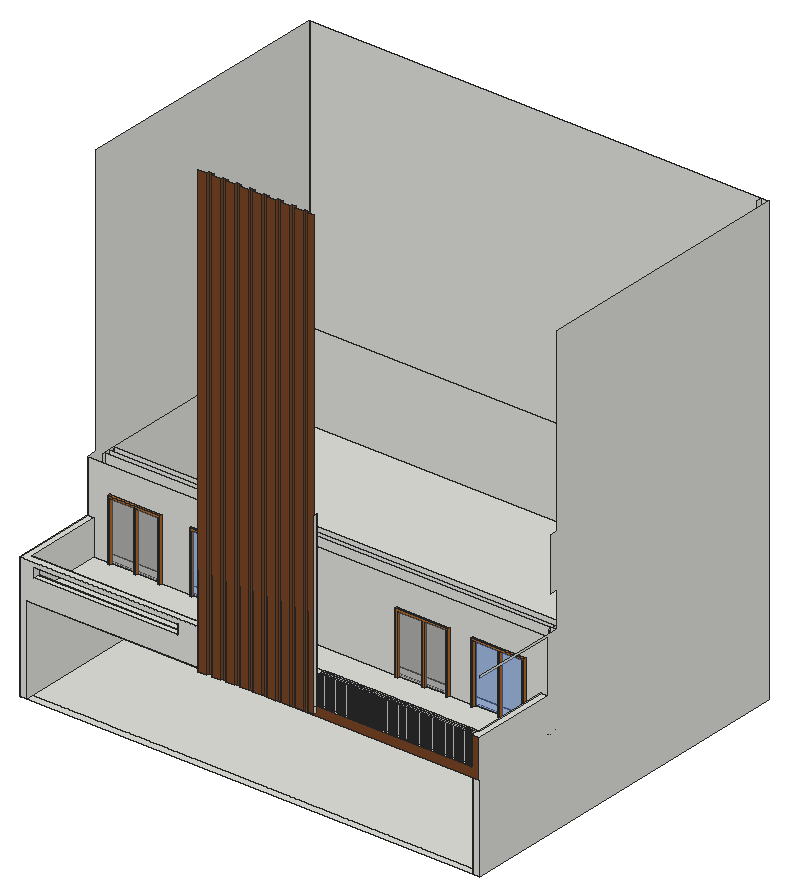
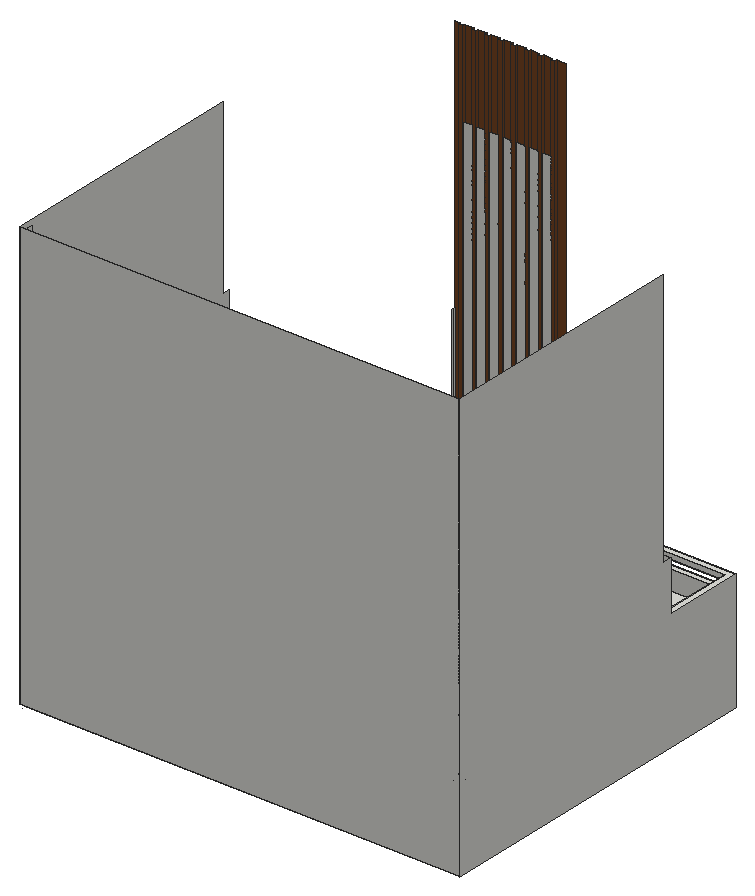
# SketchUp Ruby script. Lengths in inches.
U = 1.inch
M = Sketchup.active_model
def pt(a) = Geom::Point3d.new(a.map { |v| v * U })
def face(e, loops, mat)
  f = e.add_face(loops[0].map { |a| pt(a) })
  loops[1..].each { |l| e.add_face(l.map { |a| pt(a) }).erase! }
  f.material = f.back_material = mat if mat
  f
end
# faces: each face lists its corners as indices into pts; further lists are holes
def faces(e, pts, list, mat = nil) = list.each { |f| face(e, (f[0].is_a?(Array) ? f : [f]).map { |l| l.map { |i| pts[i] } }, mat) }
# xy, xz, yz: faces in a plane at the given z, y or x. An outline is a flat list of corners, or four numbers for a rectangle; further outlines are holes
def ring(l) = l.size == 4 ? [[l[0], l[1]], [l[2], l[1]], [l[2], l[3]], [l[0], l[3]]] : l.each_slice(2).to_a
def flat(e, list, mat, &to3) = list.each { |f| face(e, (f[0].is_a?(Array) ? f : [f]).map { |l| ring(l).map { |u, v| to3.(u, v) } }, mat) }
def xy(e, z, list, mat = nil) = flat(e, list, mat) { |x, y| [x, y, z] }
def xz(e, y, list, mat = nil) = flat(e, list, mat) { |x, z| [x, y, z] }
def yz(e, x, list, mat = nil) = flat(e, list, mat) { |y, z| [x, y, z] }
def lines(e, pts, list) = list.each { |a, b| e.add_line(pt(pts[a]), pt(pts[b])) }
# prism: a flat outline (further loops are holes) pulled along v
def prism(e, loops, v, mat = nil)
  f = face(e, loops, mat); d = Geom::Vector3d.new(v.map { |x| x * U })
  f.pushpull(f.normal.samedirection?(d) ? d.length : -d.length)
end
def box(e, o, s, mat = nil) = prism(e, [[o, [o[0] + s[0], o[1], o[2]], [o[0] + s[0], o[1] + s[1], o[2]], [o[0], o[1] + s[1], o[2]]]], [0, 0, s[2]], mat)
def at(x, y, z, deg = 0) = Geom::Transformation.translation(pt([x, y, z])) * Geom::Transformation.rotation(ORIGIN, Z_AXIS, deg.degrees)
def axes(o, x, y, z) = Geom::Transformation.new([*x, 0, *y, 0, *z, 0, *pt(o).to_a, 1])
def part(name) = M.definitions.add(name)
# library, detail: a bought-in or finely detailed component or shape, given as its bounding box
def library(name, o, s) = part(name).tap { |d| box(d.entities, o, s) }
def detail(e, o, s) = box(e.add_group.entities, o, s)
def put(e, d, t, mat = nil) = e.add_instance(d, t).tap { |i| i.material = mat if mat }
def group(e, t, mat = nil) = e.add_group.tap { |g| g.transformation = t; g.material = mat if mat }.entities
root = M.entities
M.materials.add("[Translucent Glass Blue]").color = [100, 149, 237]
M.materials["[Translucent Glass Blue]"].alpha = 0.5
M.materials.add("[Translucent Glass Gray]").color = [128, 128, 128]
M.materials["[Translucent Glass Gray]"].alpha = 0.5
M.materials.add("[Wood Bamboo]").color = [177, 105, 43]
M.materials.add("[Wood Veneer 01]").color = [120, 70, 37]
xy(root,0,[[0,6,1.4375,499.375],[1.4375,6,2.375,499.375],[2.375,6,2.375,499.375,620.5,499.375,620.5,490.375,9,490.375,9,6],[9,6,620.5,15],[620.5,6,620.75,497.0625],
  [620.75,6,628.8125,490.375],[628.8125,6,629.5625,499.375],[629.5625,6,630,499.375],[9,15,620.5,490.375],[620.75,490.375,628.8125,499.375],
  [620.5,497.0625,620.75,499.3125],[620.5,499.3125,620.75,499.375]])
xy(root,120,[[248.625,0,248.625,6,406.875,6,406.875,3,261.1,3,261.1,0],[406.875,3,406.875,6,9,6,9,490.375,620.5,490.375,620.5,3],[620.5,3,630,6]])
xy(root,120.375,[[267.4375,0,279.91,3]])
xy(root,120.75,[[286.25,0,298.72,3]])
xy(root,121.125,[[305.06,0,317.53,3]])
xy(root,121.5,[[323.87,0,336.34,3]])
xy(root,121.875,[[342.68,0,355.16,3]])
xy(root,122.0625,[[621,125.83,628.8125,136.3125]])
xy(root,122.25,[[361.49,0,373.97,3]])
xy(root,122.625,[[380.31,0,392.78,3]])
xy(root,123,[[399.12,0,406.875,3],[9,15,621,15,621,121.57,599.4,121.57,599.4,118.57,596.4,118.57,596.4,121.57,567.09,121.57,567.09,118.57,563.4,118.57,563.4,123.19,530.4,123.19,530.4,118.57,527.4,118.57,527.4,121.57,495.49,121.57,495.49,118.57,492.49,118.57,492.49,121.57,463.62,121.57,463.62,118.57,459.49,118.57,459.49,121.57,426.49,121.57,426.49,118.57,423.49,118.57,423.49,121.57,213.64,121.57,213.64,118.57,210.64,118.57,210.64,121.57,180.6,121.57,180.6,118.57,177.64,118.57,177.64,121.57,144.64,121.57,144.64,118.57,141.64,118.57,141.64,121.57,101.8,121.57,101.8,118.57,98.8,118.57,98.8,121.57,68.43,121.57,68.43,118.57,65.8,118.57,65.8,121.57,32.8,121.57,32.8,118.57,29.8,118.57,29.8,121.57,9,121.57],[423.49,118.57,426.49,121.57],[459.49,118.57,463.62,121.57],[492.49,118.57,495.49,121.57],
  [527.4,118.57,530.4,121.57],[563.4,118.57,567.09,121.57],[596.4,118.57,599.4,121.57],[620.5,121.57,621,125.58],[0,125.58,619.6875,125.83],
  [619.6875,125.58,620.5,125.83],[620.5,125.58,621,125.83],[621,125.58,628.8125,125.83],[620.5,125.83,621,135.01],[621,125.83,628.8125,135.01],
  [620.5,135.01,621,136.3125],[621,135.01,628.8125,136.3125],[620.5,136.3125,621,139.19],[9,139.19,620.5,146.07],[620.5,139.19,621,146.07],
  [9,146.07,620.5,155.08],[620.5,146.07,621,155.08],[9,155.08,621,490.375]])
xy(root,123.125,[[621,125.83,628.8125,135.01],[621,135.01,628.8125,136.3125]])
xy(root,132.4,[[406.875,3,620.5,3,620.5,6,618.8,6,618.8,15,617.26,15,617.26,6,615.74,6,615.74,15,614.19,15,614.19,6,612.68,6,612.68,15,611.13,15,611.13,6,609.62,6,609.62,15,608.07,15,608.07,6,606.55,6,606.55,15,605.01,15,605.01,6,603.49,6,603.49,15,601.94,15,601.94,6,600.43,6,600.43,15,598.88,15,598.88,6,597.37,6,597.37,15,595.82,15,595.82,6.5,594.3,6.5,594.3,15,592.76,15,592.76,6,590.74,6,590.74,15,589.19,15,589.19,6,587.18,6,587.18,15,585.63,15,585.63,6,583.62,6,583.62,15,582.07,15,582.07,6,580.05,6,580.05,15,578.51,15,578.51,6,576.49,6,576.49,15,574.94,15,574.94,6,572.93,6,572.93,15,571.38,15,571.38,6,569.37,6,569.37,15,567.82,15,567.82,6,565.8,6,565.8,15,564.26,15,564.26,6,562.24,6,562.24,15,560.69,15,560.69,6,558.68,6,558.68,15,557.13,15,557.13,6,555.12,6,555.12,15,553.57,15,553.57,6,551.55,6,551.55,15,550.01,15,550.01,6,547.99,6,547.99,15,546.44,15,546.44,6,544.43,6,544.43,15,542.88,15,542.88,6,540.87,6,540.87,15,539.32,15,539.32,6,537.3,6,537.3,15,535.76,15,535.76,6,533.74,6,533.74,15,532.19,15,532.19,6,530.18,6,530.18,15,528.63,15,528.63,6,526.62,6,526.62,15,525.07,15,525.07,6,523.05,6,523.05,15,521.51,15,521.51,6,519.3,6,519.3,15,517.76,15,517.76,6,515.55,6,515.55,15,514.01,15,514.01,6,511.8,6,511.8,15,510.26,15,510.26,6,508.05,6,508.05,15,506.51,15,506.51,6,504.3,6,504.3,15,502.76,15,502.76,6,500.55,6,500.55,15,499.01,15,499.01,6,496.8,6,496.8,15,495.26,15,495.26,6,493.05,6,493.05,15,491.51,15,491.51,6,489.3,6,489.3,15,487.76,15,487.76,6,485.55,6,485.55,15,484.01,15,484.01,6,481.8,6,481.8,15,480.26,15,480.26,6,478.05,6,478.05,15,476.51,15,476.51,6,474.3,6,474.3,15,472.76,15,472.76,6,470.55,6,470.55,15,469.01,15,469.01,6,466.8,6,466.8,15,465.26,15,465.26,6,463.05,6,463.05,15,461.51,15,461.51,6,459.3,6,459.3,15,457.76,15,457.76,6,455.55,6,455.55,15,454.01,15,454.01,6,451.8,6,451.8,15,450.26,15,450.26,6,448.05,6,448.05,15,446.51,15,446.51,6,444.3,6,444.3,15,442.76,15,442.76,6,440.55,6,440.55,15,439.01,15,439.01,6,436.8,6,436.8,15,435.26,15,435.26,6,433.05,6,433.05,15,431.51,15,431.51,6,429.3,6,429.3,15,427.76,15,427.76,6,425.55,6,425.55,15,424.01,15,424.01,6,421.8,6,421.8,15,420.26,15,420.26,6,418.05,6,418.05,15,416.51,15,416.51,6,414.3,6,414.3,15,412.76,15,412.76,6,410.55,6,410.55,15,409.01,15,409.01,6,406.875,6]])
xy(root,150.64,[[18.24,6,215.68,15]])
xy(root,164.2,[[18.24,6,215.68,15]])
xy(root,171,[[620.5,3,630,3,630,121.92,621,121.57,621,15,618.8,15,618.8,6,620.5,6],[0,6,409.01,6,409.01,15,9,15,9,121.57,0,121.57],[410.55,6,412.76,15],[414.3,6,416.51,15],[418.05,6,420.26,15],
  [421.8,6,424.01,15],[425.55,6,427.76,15],[429.3,6,431.51,15],[433.05,6,435.26,15],[436.8,6,439.01,15],
  [440.55,6,442.76,15],[444.3,6,446.51,15],[448.05,6,450.26,15],[451.8,6,454.01,15],[455.55,6,457.76,15],
  [459.3,6,461.51,15],[463.05,6,465.26,15],[466.8,6,469.01,15],[470.55,6,472.76,15],[474.3,6,476.51,15],
  [478.05,6,480.26,15],[481.8,6,484.01,15],[485.55,6,487.76,15],[489.3,6,491.51,15],[493.05,6,495.26,15],
  [496.8,6,499.01,15],[500.55,6,502.76,15],[504.3,6,506.51,15],[508.05,6,510.26,15],[511.8,6,514.01,15],
  [515.55,6,517.76,15],[519.3,6,521.51,15],[523.05,6,525.07,15],[526.62,6,528.63,15],[530.18,6,532.19,15],
  [533.74,6,535.76,15],[537.3,6,539.32,15],[540.87,6,542.88,15],[544.43,6,546.44,15],[547.99,6,550.01,15],
  [551.55,6,553.57,15],[555.12,6,557.13,15],[558.68,6,560.69,15],[562.24,6,564.26,15],[565.8,6,567.82,15],
  [569.37,6,571.38,15],[572.93,6,574.94,15],[576.49,6,578.51,15],[580.05,6,582.07,15],[583.62,6,585.63,15],
  [587.18,6,589.19,15],[590.74,6,592.76,15],[597.37,6,598.88,15],[600.43,6,601.94,15],[603.49,6,605.01,15],
  [606.55,6,608.07,15],[609.62,6,611.13,15],[612.68,6,614.19,15],[615.74,6,617.26,15],[594.3,6.5,595.82,15]])
xy(root,204,[[32.8,118.57,65.8,121.57],[68.43,118.57,98.8,121.57],[144.64,118.57,177.64,121.57],[180.6,118.57,210.64,121.57],[426.49,118.57,459.49,121.57],
  [463.62,118.57,492.49,121.57],[530.4,118.57,563.4,121.57],[567.09,118.57,596.4,121.57],[530.4,121.57,563.4,123.19]],"[Wood Bamboo]")
xy(root,207,[[29.8,118.57,101.8,121.57],[141.64,118.57,213.64,121.57],[423.49,118.57,495.49,121.57],[527.4,118.57,599.4,121.57]],"[Wood Bamboo]")
xz(root,0,[[248.625,120,261.1,735.4375],[267.4375,120.375,279.91,735.4375],[286.25,120.75,298.72,735.4375],[305.06,121.125,317.53,735.4375],[323.87,121.5,336.34,735.4375],
  [342.68,121.875,355.16,735.4375],[361.49,122.25,373.97,735.4375],[380.31,122.625,392.78,735.21],[399.12,123,406.875,735.4375]],"[Wood Veneer 01]")
xz(root,3,[[267.4375,120.375,279.91,612],[286.25,120.75,298.72,612],[305.06,121.125,317.53,612],[323.87,121.5,336.34,612],[342.68,121.875,355.16,612],
  [361.49,122.25,373.97,612],[380.31,122.625,392.78,612]])
xz(root,3,[[261.1,120,630,120,630,171,620.5,171,620.5,132.4,406.875,132.4,406.875,123,399.12,123,399.12,735.4375,392.78,735.4375,392.78,122.625,380.31,122.625,380.31,735.4375,373.97,735.4375,373.97,122.25,361.49,122.25,361.49,735.4375,355.16,735.4375,355.16,121.875,342.68,121.875,342.68,735.4375,336.34,735.4375,336.34,121.5,323.87,121.5,323.87,735.4375,317.53,735.4375,317.53,121.125,305.06,121.125,305.06,735.4375,298.72,735.4375,298.72,120.75,286.25,120.75,286.25,735.4375,279.91,735.4375,279.91,120.375,267.4375,120.375,267.4375,735.4375,261.1,735.4375]],"[Wood Veneer 01]")
xz(root,6,[[[0,0,9,0,9,120,248.625,120,248.625,171,0,171],[18.24,150.64,215.68,164.2]],[620.5,0,630,120],[248.625,120,406.875,123],[248.625,123,406.875,171],[406.875,132.4,409.01,171],
  [410.55,132.4,412.76,171],[414.3,132.4,416.51,171],[418.05,132.4,420.26,171],[421.8,132.4,424.01,171],[425.55,132.4,427.76,171],
  [429.3,132.4,431.51,171],[433.05,132.4,435.26,171],[436.8,132.4,439.01,171],[440.55,132.4,442.76,171],[444.3,132.4,446.51,171],
  [448.05,132.4,450.26,171],[451.8,132.4,454.01,171],[455.55,132.4,457.76,171],[459.3,132.4,461.51,171],[463.05,132.4,465.26,171],
  [466.8,132.4,469.01,171],[470.55,132.4,472.76,171],[474.3,132.4,476.51,171],[478.05,132.4,480.26,171],[481.8,132.4,484.01,171],
  [485.55,132.4,487.76,171],[489.3,132.4,491.51,171],[493.05,132.4,495.26,171],[496.8,132.4,499.01,171],[500.55,132.4,502.76,171],
  [504.3,132.4,506.51,171],[508.05,132.4,510.26,171],[511.8,132.4,514.01,171],[515.55,132.4,517.76,171],[519.3,132.4,521.51,171],
  [523.05,132.4,525.07,171],[526.62,132.4,528.63,171],[530.18,132.4,532.19,171],[533.74,132.4,535.76,171],[537.3,132.4,539.32,171],
  [540.87,132.4,542.88,171],[544.43,132.4,546.44,171],[547.99,132.4,550.01,171],[551.55,132.4,553.57,171],[555.12,132.4,557.13,171],
  [558.68,132.4,560.69,171],[562.24,132.4,564.26,171],[565.8,132.4,567.82,171],[569.37,132.4,571.38,171],[572.93,132.4,574.94,171],
  [576.49,132.4,578.51,171],[580.05,132.4,582.07,171],[583.62,132.4,585.63,171],[587.18,132.4,589.19,171],[590.74,132.4,592.76,171],
  [597.37,132.4,598.88,171],[600.43,132.4,601.94,171],[603.49,132.4,605.01,171],[606.55,132.4,608.07,171],[609.62,132.4,611.13,171],
  [612.68,132.4,614.19,171],[615.74,132.4,617.26,171],[618.8,132.4,620.32,171],[620.32,132.4,620.5,171],[248.625,171,406.875,243]])
xz(root,6.5,[[594.3,132.4,595.82,171]])
xz(root,15,[[620.5,122.75,621,122.9375],[620.5,122.9375,621,123],[[9,123,9,171,409.01,171,409.01,132.4,410.55,132.4,410.55,171,412.76,171,412.76,132.4,414.3,132.4,414.3,171,416.51,171,416.51,132.4,418.05,132.4,418.05,171,420.26,171,420.26,132.4,421.8,132.4,421.8,171,424.01,171,424.01,132.4,425.55,132.4,425.55,171,427.76,171,427.76,132.4,429.3,132.4,429.3,171,431.51,171,431.51,132.4,433.05,132.4,433.05,171,435.26,171,435.26,132.4,436.8,132.4,436.8,171,439.01,171,439.01,132.4,440.55,132.4,440.55,171,442.76,171,442.76,132.4,444.3,132.4,444.3,171,446.51,171,446.51,132.4,448.05,132.4,448.05,171,450.26,171,450.26,132.4,451.8,132.4,451.8,171,454.01,171,454.01,132.4,455.55,132.4,455.55,171,457.76,171,457.76,132.4,459.3,132.4,459.3,171,461.51,171,461.51,132.4,463.05,132.4,463.05,171,465.26,171,465.26,132.4,466.8,132.4,466.8,171,469.01,171,469.01,132.4,470.55,132.4,470.55,171,472.76,171,472.76,132.4,474.3,132.4,474.3,171,476.51,171,476.51,132.4,478.05,132.4,478.05,171,480.26,171,480.26,132.4,481.8,132.4,481.8,171,484.01,171,484.01,132.4,485.55,132.4,485.55,171,487.76,171,487.76,132.4,489.3,132.4,489.3,171,491.51,171,491.51,132.4,493.05,132.4,493.05,171,495.26,171,495.26,132.4,496.8,132.4,496.8,171,499.01,171,499.01,132.4,500.55,132.4,500.55,171,502.76,171,502.76,132.4,504.3,132.4,504.3,171,506.51,171,506.51,132.4,508.05,132.4,508.05,171,510.26,171,510.26,132.4,511.8,132.4,511.8,171,514.01,171,514.01,132.4,515.55,132.4,515.55,171,517.76,171,517.76,132.4,519.3,132.4,519.3,171,521.51,171,521.51,132.4,523.05,132.4,523.05,171,525.07,171,525.07,132.4,526.62,132.4,526.62,171,528.63,171,528.63,132.4,530.18,132.4,530.18,171,532.19,171,532.19,132.4,533.74,132.4,533.74,171,535.76,171,535.76,132.4,537.3,132.4,537.3,171,539.32,171,539.32,132.4,540.87,132.4,540.87,171,542.88,171,542.88,132.4,544.43,132.4,544.43,171,546.44,171,546.44,132.4,547.99,132.4,547.99,171,550.01,171,550.01,132.4,551.55,132.4,551.55,171,553.57,171,553.57,132.4,555.12,132.4,555.12,171,557.13,171,557.13,132.4,558.68,132.4,558.68,171,560.69,171,560.69,132.4,562.24,132.4,562.24,171,564.26,171,564.26,132.4,565.8,132.4,565.8,171,567.82,171,567.82,132.4,569.37,132.4,569.37,171,571.38,171,571.38,132.4,572.93,132.4,572.93,171,574.94,171,574.94,132.4,576.49,132.4,576.49,171,578.51,171,578.51,132.4,580.05,132.4,580.05,171,582.07,171,582.07,132.4,583.62,132.4,583.62,171,585.63,171,585.63,132.4,587.18,132.4,587.18,171,589.19,171,589.19,132.4,590.74,132.4,590.74,171,592.76,171,592.76,132.4,594.3,132.4,594.3,171,595.82,171,595.82,132.4,597.37,132.4,597.37,171,598.88,171,598.88,132.4,600.43,132.4,600.43,171,601.94,171,601.94,132.4,603.49,132.4,603.49,171,605.01,171,605.01,132.4,606.55,132.4,606.55,171,608.07,171,608.07,132.4,609.62,132.4,609.62,171,611.13,171,611.13,132.4,612.68,132.4,612.68,171,614.19,171,614.19,132.4,615.74,132.4,615.74,171,617.26,171,617.26,132.4,618.8,132.4,618.8,171,620.5,171,620.5,123],[18.24,150.64,215.68,164.2]],[620.5,123,621,171]])
xz(root,118.57,[[29.8,123,32.8,123,32.8,204,65.8,204,65.8,123,68.43,123,68.43,204,98.8,204,98.8,123,101.8,123,101.8,207,29.8,207],[141.64,123,144.64,123,144.64,204,177.64,204,177.64,123,180.6,123,180.6,204,210.64,204,210.64,123,213.64,123,213.64,207,141.64,207],[423.49,123,426.49,123,426.49,204,459.49,204,459.49,123,463.62,123,463.62,204,492.49,204,492.49,123,495.49,123,495.49,207,423.49,207],[527.4,123,530.4,123,530.4,204,563.4,204,563.4,123,567.09,123,567.09,204,596.4,204,596.4,123,599.4,123,599.4,207,527.4,207]],"[Wood Bamboo]")
xz(root,121.57,[[9,123,29.8,123,29.8,207,101.8,207,101.8,123,141.64,123,141.64,207,213.64,207,213.64,123,423.49,123,423.49,207,495.49,207,495.49,123,527.4,123,527.4,207,599.4,207,599.4,123,621,123,621,123.125,630,123.125,630,243,0,243,0,171,9,171],[423.49,123,423.49,207,495.49,207,495.49,123,492.49,123,492.49,204,463.62,204,463.62,123,459.49,123,459.49,204,426.49,204,426.49,123]])
xz(root,121.57,[[144.64,123,177.64,204],[180.6,123,210.64,204],[567.09,123,596.4,204]],"[Translucent Glass Blue]")
xz(root,121.57,[[32.8,123,65.8,204],[68.43,123,98.8,204],[426.49,123,459.49,204],[463.62,123,492.49,204]],"[Translucent Glass Gray]")
xz(root,121.57,[[527.4,123,527.4,207,599.4,207,599.4,123,596.4,123,596.4,204,567.09,204,567.09,123,563.4,123,563.4,204,530.4,204,530.4,123]],"[Wood Bamboo]")
xz(root,123.19,[[530.4,123,563.4,204]],"[Translucent Glass Blue]")
xz(root,125.58,[[621,123,628.8125,123.125],[621,123.125,628.8125,123.1875]])
xz(root,125.83,[[619.6875,122.0625,619.6875,123,620.5,123,620.5,122.9375,621,122.9375,621,122.0625],[621,122.0625,628.8125,123],[620.5,122.9375,621,123],[621,123,628.8125,123.125]])
xz(root,136.3125,[[621,122.0625,628.8125,123],[620.5,123,621,125.6875],[621,123,628.8125,123.125],[621,123.125,621,125.6875,620.5,125.6875,620.5,246,628.8125,246,628.8125,123.125]])
xz(root,139.19,[[9,123,621,243]])
xz(root,146.07,[[9,123,621,243]])
xz(root,155.08,[[9,123,621,243]])
xz(root,490.375,[[9,0,620.5,120],[620.75,0,628.8125,0,628.8125,243,621,243,621,123,620.75,123],[9,123,620.75,243],[620.75,123,621,243]])
xz(root,497.0625,[[620.5,0,620.75,612]])
xz(root,499.375,[[0,0,1.4375,612],[1.4375,0,2.375,612],[2.375,0,629.5625,612],[629.5625,0,630,122.0625],[629.5625,122.0625,630,123],
  [629.5625,123,630,612]])
yz(root,0,[[6,0,6,171,121.57,171,121.57,243,136.3125,243,136.3125,612,499.375,612,499.375,0]])
yz(root,9,[[6,0,490.375,120],[15,123,121.57,171],[136.3125,123,139.19,243],[139.19,123,146.07,243],[146.07,123,155.08,243],
  [155.08,123,490.375,243]])
yz(root,18.24,[[6,150.64,15,164.2]])
yz(root,29.8,[[118.57,123,121.57,207]],"[Wood Bamboo]")
yz(root,32.8,[[118.57,123,121.57,204]],"[Wood Bamboo]")
yz(root,65.8,[[118.57,123,121.57,204]],"[Wood Bamboo]")
yz(root,68.43,[[118.57,123,121.57,204]],"[Wood Bamboo]")
yz(root,98.8,[[118.57,123,121.57,204]],"[Wood Bamboo]")
yz(root,101.8,[[118.57,123,121.57,207]],"[Wood Bamboo]")
yz(root,141.64,[[118.57,123,121.57,207]],"[Wood Bamboo]")
yz(root,144.64,[[118.57,123,121.57,204]],"[Wood Bamboo]")
yz(root,177.64,[[118.57,123,121.57,204]],"[Wood Bamboo]")
yz(root,180.6,[[118.57,123,121.57,204]],"[Wood Bamboo]")
yz(root,210.64,[[118.57,123,121.57,204]],"[Wood Bamboo]")
yz(root,213.64,[[118.57,123,121.57,207]],"[Wood Bamboo]")
yz(root,215.68,[[6,150.64,15,164.2]])
yz(root,248.625,[[0,120,6,243]])
yz(root,261.1,[[0,120,3,735.4375]],"[Wood Veneer 01]")
yz(root,267.4375,[[0,120.375,3,243.375]])
yz(root,279.91,[[0,120.375,3,735.4375]],"[Wood Veneer 01]")
yz(root,286.25,[[0,120.75,3,243.75]])
yz(root,298.72,[[0,120.75,3,735.4375]],"[Wood Veneer 01]")
yz(root,305.06,[[0,121.125,3,244.125]])
yz(root,317.53,[[0,121.125,3,735.4375]],"[Wood Veneer 01]")
yz(root,323.87,[[0,121.5,3,244.5]])
yz(root,336.34,[[0,121.5,3,735.4375]],"[Wood Veneer 01]")
yz(root,342.68,[[0,121.875,3,244.875]])
yz(root,355.16,[[0,121.875,3,735.4375]],"[Wood Veneer 01]")
yz(root,361.49,[[0,122.25,3,245.25]])
yz(root,373.97,[[0,122.25,3,735.4375]],"[Wood Veneer 01]")
yz(root,380.31,[[0,122.625,3,245.625]])
yz(root,392.78,[[0,122.625,3,735.21]],"[Wood Veneer 01]")
yz(root,399.12,[[0,123,3,246]])
yz(root,406.875,[[0,123,3,132.4],[3,123,6,132.4],[0,132.4,3,366.375],[3,132.4,6,366.375]])
yz(root,409.01,[[6,132.4,15,171]])
yz(root,410.55,[[6,132.4,15,171]])
yz(root,412.76,[[6,132.4,15,171]])
yz(root,414.3,[[6,132.4,15,171]])
yz(root,416.51,[[6,132.4,15,171]])
yz(root,418.05,[[6,132.4,15,171]])
yz(root,420.26,[[6,132.4,15,171]])
yz(root,421.8,[[6,132.4,15,171]])
yz(root,423.49,[[118.57,123,121.57,207]],"[Wood Bamboo]")
yz(root,424.01,[[6,132.4,15,171]])
yz(root,425.55,[[6,132.4,15,171]])
yz(root,426.49,[[118.57,123,121.57,204]],"[Wood Bamboo]")
yz(root,427.76,[[6,132.4,15,171]])
yz(root,429.3,[[6,132.4,15,171]])
yz(root,431.51,[[6,132.4,15,171]])
yz(root,433.05,[[6,132.4,15,171]])
yz(root,435.26,[[6,132.4,15,171]])
yz(root,436.8,[[6,132.4,15,171]])
yz(root,439.01,[[6,132.4,15,171]])
yz(root,440.55,[[6,132.4,15,171]])
yz(root,442.76,[[6,132.4,15,171]])
yz(root,444.3,[[6,132.4,15,171]])
yz(root,446.51,[[6,132.4,15,171]])
yz(root,448.05,[[6,132.4,15,171]])
yz(root,450.26,[[6,132.4,15,171]])
yz(root,451.8,[[6,132.4,15,171]])
yz(root,454.01,[[6,132.4,15,171]])
yz(root,455.55,[[6,132.4,15,171]])
yz(root,457.76,[[6,132.4,15,171]])
yz(root,459.3,[[6,132.4,15,171]])
yz(root,459.49,[[118.57,123,121.57,204]],"[Wood Bamboo]")
yz(root,461.51,[[6,132.4,15,171]])
yz(root,463.05,[[6,132.4,15,171]])
yz(root,463.62,[[118.57,123,121.57,204]],"[Wood Bamboo]")
yz(root,465.26,[[6,132.4,15,171]])
yz(root,466.8,[[6,132.4,15,171]])
yz(root,469.01,[[6,132.4,15,171]])
yz(root,470.55,[[6,132.4,15,171]])
yz(root,472.76,[[6,132.4,15,171]])
yz(root,474.3,[[6,132.4,15,171]])
yz(root,476.51,[[6,132.4,15,171]])
yz(root,478.05,[[6,132.4,15,171]])
yz(root,480.26,[[6,132.4,15,171]])
yz(root,481.8,[[6,132.4,15,171]])
yz(root,484.01,[[6,132.4,15,171]])
yz(root,485.55,[[6,132.4,15,171]])
yz(root,487.76,[[6,132.4,15,171]])
yz(root,489.3,[[6,132.4,15,171]])
yz(root,491.51,[[6,132.4,15,171]])
yz(root,492.49,[[118.57,123,121.57,204]],"[Wood Bamboo]")
yz(root,493.05,[[6,132.4,15,171]])
yz(root,495.26,[[6,132.4,15,171]])
yz(root,495.49,[[118.57,123,121.57,207]],"[Wood Bamboo]")
yz(root,496.8,[[6,132.4,15,171]])
yz(root,499.01,[[6,132.4,15,171]])
yz(root,500.55,[[6,132.4,15,171]])
yz(root,502.76,[[6,132.4,15,171]])
yz(root,504.3,[[6,132.4,15,171]])
yz(root,506.51,[[6,132.4,15,171]])
yz(root,508.05,[[6,132.4,15,171]])
yz(root,510.26,[[6,132.4,15,171]])
yz(root,511.8,[[6,132.4,15,171]])
yz(root,514.01,[[6,132.4,15,171]])
yz(root,515.55,[[6,132.4,15,171]])
yz(root,517.76,[[6,132.4,15,171]])
yz(root,519.3,[[6,132.4,15,171]])
yz(root,521.51,[[6,132.4,15,171]])
yz(root,523.05,[[6,132.4,15,171]])
yz(root,525.07,[[6,132.4,15,171]])
yz(root,526.62,[[6,132.4,15,171]])
yz(root,527.4,[[118.57,123,121.57,207]])
yz(root,528.63,[[6,132.4,15,171]])
yz(root,530.18,[[6,132.4,15,171]])
yz(root,530.4,[[118.57,123,121.57,204],[121.57,123,123.19,204]],"[Wood Bamboo]")
yz(root,532.19,[[6,132.4,15,171]])
yz(root,533.74,[[6,132.4,15,171]])
yz(root,535.76,[[6,132.4,15,171]])
yz(root,537.3,[[6,132.4,15,171]])
yz(root,539.32,[[6,132.4,15,171]])
yz(root,540.87,[[6,132.4,15,171]])
yz(root,542.88,[[6,132.4,15,171]])
yz(root,544.43,[[6,132.4,15,171]])
yz(root,546.44,[[6,132.4,15,171]])
yz(root,547.99,[[6,132.4,15,171]])
yz(root,550.01,[[6,132.4,15,171]])
yz(root,551.55,[[6,132.4,15,171]])
yz(root,553.57,[[6,132.4,15,171]])
yz(root,555.12,[[6,132.4,15,171]])
yz(root,557.13,[[6,132.4,15,171]])
yz(root,558.68,[[6,132.4,15,171]])
yz(root,560.69,[[6,132.4,15,171]])
yz(root,562.24,[[6,132.4,15,171]])
yz(root,563.4,[[118.57,123,121.57,204],[121.57,123,123.19,204]],"[Wood Bamboo]")
yz(root,564.26,[[6,132.4,15,171]])
yz(root,565.8,[[6,132.4,15,171]])
yz(root,567.09,[[118.57,123,121.57,204]],"[Wood Bamboo]")
yz(root,567.82,[[6,132.4,15,171]])
yz(root,569.37,[[6,132.4,15,171]])
yz(root,571.38,[[6,132.4,15,171]])
yz(root,572.93,[[6,132.4,15,171]])
yz(root,574.94,[[6,132.4,15,171]])
yz(root,576.49,[[6,132.4,15,171]])
yz(root,578.51,[[6,132.4,15,171]])
yz(root,580.05,[[6,132.4,15,171]])
yz(root,582.07,[[6,132.4,15,171]])
yz(root,583.62,[[6,132.4,15,171]])
yz(root,585.63,[[6,132.4,15,171]])
yz(root,587.18,[[6,132.4,15,171]])
yz(root,589.19,[[6,132.4,15,171]])
yz(root,590.74,[[6,132.4,15,171]])
yz(root,592.76,[[6,132.4,15,171]])
yz(root,594.3,[[6.5,132.4,15,171]])
yz(root,595.82,[[6.5,132.4,15,171]])
yz(root,596.4,[[118.57,123,121.57,204]],"[Wood Bamboo]")
yz(root,597.37,[[6,132.4,15,171]])
yz(root,598.88,[[6,132.4,15,171]])
yz(root,599.4,[[118.57,123,121.57,207]],"[Wood Bamboo]")
yz(root,600.43,[[6,132.4,15,171]])
yz(root,601.94,[[6,132.4,15,171]])
yz(root,603.49,[[6,132.4,15,171]])
yz(root,605.01,[[6,132.4,15,171]])
yz(root,606.55,[[6,132.4,15,171]])
yz(root,608.07,[[6,132.4,15,171]])
yz(root,609.62,[[6,132.4,15,171]])
yz(root,611.13,[[6,132.4,15,171]])
yz(root,612.68,[[6,132.4,15,171]])
yz(root,614.19,[[6,132.4,15,171]])
yz(root,615.74,[[6,132.4,15,171]])
yz(root,617.26,[[6,132.4,15,171]])
yz(root,618.8,[[6,132.4,15,171]])
yz(root,620.5,[[6,0,490.375,120],[3,132.4,6,169.8125],[3,169.8125,6,171]])
yz(root,620.75,[[490.375,0,497.0625,612]])
yz(root,621,[[15,122.0625,125.83,122.9375],[125.83,122.0625,135.01,123],[135.01,122.0625,136.3125,123],[15,122.9375,125.83,123],[15,123,121.57,171],
  [121.57,123,125.58,123.125],[125.58,123,125.83,123.125],[125.83,123,135.01,123.125],[135.01,123,136.3125,123.125],[136.3125,123,136.94,243],
  [136.94,123,139.19,243],[139.19,123,146.07,243],[146.07,123,155.08,243],[155.08,123,490.375,243],[121.57,123.125,125.58,123.1875],
  [135.01,123.125,136.3125,243]])
yz(root,628.8125,[[125.83,122.0625,136.3125,123],[125.83,123,136.3125,123.125],[125.83,123.125,136.3125,123.3125]])
yz(root,630,[[6,0,499.375,0,499.375,612,136.3125,612,136.3125,366.375,126.125,366.375,126.125,294.0625,136.3125,294.0625,136.3125,246,126.125,246,126.125,245.8125,6,245.8125,6,243,121.57,243,121.57,171,3,171,3,120,6,120]])
p = [[630,121.92,123],[621,121.57,123],[621,121.57,123.125],[621,121.57,123.1875],[630,121.92,123.1875],[630,121.92,123.125],
  [9,490.375,120],[0,490.375,120],[9,499.375,120],[621,6,122.0625],[621,15,122.0625],[628.8125,6,122.0625],
  [628.8125,125.83,122.0625],[630,125.83,122.0625],[620.75,506,0],[620.5,506,0],[628.8125,125.83,123.3125],[628.8125,125.58,123.3125],
  [629.5625,125.83,123.3125],[629.5625,125.58,123.3125],[629.5625,125.83,123.125],[629.5625,125.58,123.125],[628.8125,125.83,123],[629.5625,125.83,123],
  [619.6875,6,122.0625],[619.6875,125.83,122.0625],[628.8125,135.01,123.125],[630,135.01,123.125],[629.5625,125.58,123],[630,121.57,123.125],
  [621.87,6,132.4],[620.5,6,132.4],[624.93,6,132.4],[623.38,6,132.4],[627.99,6,132.4],[626.44,6,132.4]]
faces(root,p,[[0,1,2,3,4,5]])
lines(root,p,[[6,7],[6,8],[9,10],[11,12],[12,13],[14,15],[16,17],[18,19],[20,21],[22,23],[24,25],[26,27],
  [28,23],[5,29],[30,31],[32,33],[34,35]])
